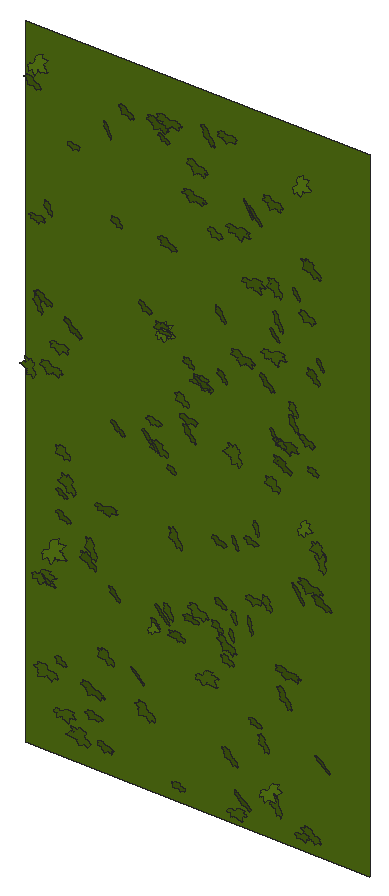
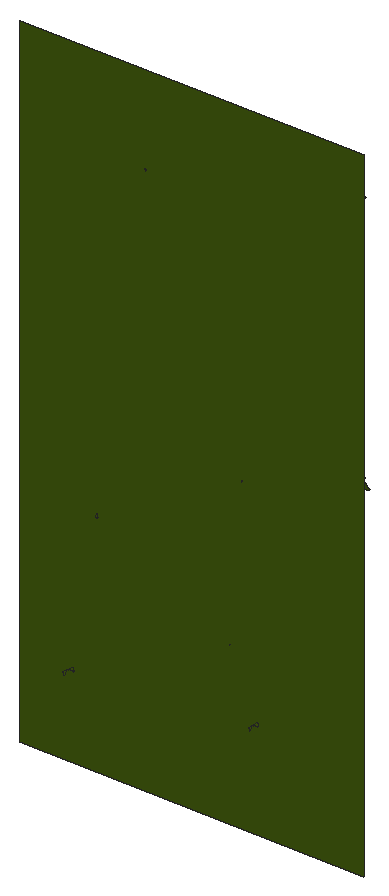
# SketchUp Ruby script. Lengths in inches.
U = 1.inch
M = Sketchup.active_model
def pt(a) = Geom::Point3d.new(a.map { |v| v * U })
def face(e, loops, mat)
  f = e.add_face(loops[0].map { |a| pt(a) })
  loops[1..].each { |l| e.add_face(l.map { |a| pt(a) }).erase! }
  f.material = f.back_material = mat if mat
  f
end
# faces: each face lists its corners as indices into pts; further lists are holes
def faces(e, pts, list, mat = nil) = list.each { |f| face(e, (f[0].is_a?(Array) ? f : [f]).map { |l| l.map { |i| pts[i] } }, mat) }
# xy, xz, yz: faces in a plane at the given z, y or x. An outline is a flat list of corners, or four numbers for a rectangle; further outlines are holes
def ring(l) = l.size == 4 ? [[l[0], l[1]], [l[2], l[1]], [l[2], l[3]], [l[0], l[3]]] : l.each_slice(2).to_a
def flat(e, list, mat, &to3) = list.each { |f| face(e, (f[0].is_a?(Array) ? f : [f]).map { |l| ring(l).map { |u, v| to3.(u, v) } }, mat) }
def xy(e, z, list, mat = nil) = flat(e, list, mat) { |x, y| [x, y, z] }
def xz(e, y, list, mat = nil) = flat(e, list, mat) { |x, z| [x, y, z] }
def yz(e, x, list, mat = nil) = flat(e, list, mat) { |y, z| [x, y, z] }
def lines(e, pts, list) = list.each { |a, b| e.add_line(pt(pts[a]), pt(pts[b])) }
# prism: a flat outline (further loops are holes) pulled along v
def prism(e, loops, v, mat = nil)
  f = face(e, loops, mat); d = Geom::Vector3d.new(v.map { |x| x * U })
  f.pushpull(f.normal.samedirection?(d) ? d.length : -d.length)
end
def box(e, o, s, mat = nil) = prism(e, [[o, [o[0] + s[0], o[1], o[2]], [o[0] + s[0], o[1] + s[1], o[2]], [o[0], o[1] + s[1], o[2]]]], [0, 0, s[2]], mat)
def at(x, y, z, deg = 0) = Geom::Transformation.translation(pt([x, y, z])) * Geom::Transformation.rotation(ORIGIN, Z_AXIS, deg.degrees)
def axes(o, x, y, z) = Geom::Transformation.new([*x, 0, *y, 0, *z, 0, *pt(o).to_a, 1])
def part(name) = M.definitions.add(name)
# library, detail: a bought-in or finely detailed component or shape, given as its bounding box
def library(name, o, s) = part(name).tap { |d| box(d.entities, o, s) }
def detail(e, o, s) = box(e.add_group.entities, o, s)
def put(e, d, t, mat = nil) = e.add_instance(d, t).tap { |i| i.material = mat if mat }
def group(e, t, mat = nil) = e.add_group.tap { |g| g.transformation = t; g.material = mat if mat }.entities
root = M.entities
M.materials.add("[Vegetation Blur 03]").color = [83, 114, 18]
c1 = part("ivy")
xy(c1.entities,0,[[0.782,0,0.786,0,0.787,0.005,0.789,0.009,0.821,0.072,0.875,0.147,1.001,0.272,1.073,0.331,1.137,0.363,1.178,0.379,1.223,0.384,1.272,0.383,1.311,0.374,1.36,0.355,1.399,0.334,1.491,0.285,1.541,0.244,1.583,0.199,1.617,0.15,1.64,0.128,1.662,0.115,1.717,0.105,1.745,0.093,1.784,0.054,1.819,0.057,1.854,0.064,1.882,0.075,1.896,0.074,1.91,0.071,1.937,0.063,1.964,0.053,1.99,0.038,2.016,0.015,2.034,0.002,2.04,0,2.038,0.003,2.036,0.007,2.033,0.038,2.036,0.068,2.045,0.1,2.055,0.116,2.064,0.123,2.077,0.129,2.088,0.129,2.106,0.132,2.118,0.13,2.179,0.132,2.207,0.133,2.225,0.133,2.242,0.138,2.22,0.162,2.207,0.186,2.206,0.213,2.212,0.236,2.228,0.262,2.247,0.274,2.298,0.283,2.355,0.294,2.37,0.296,2.376,0.295,2.377,0.3,2.377,0.303,2.385,0.329,2.411,0.37,2.426,0.392,2.449,0.407,2.511,0.426,2.561,0.444,2.619,0.466,2.589,0.469,2.561,0.476,2.501,0.5,2.449,0.516,2.424,0.523,2.401,0.535,2.377,0.556,2.372,0.568,2.36,0.575,2.268,0.586,2.225,0.592,2.207,0.599,2.194,0.61,2.143,0.65,2.13,0.664,2.122,0.682,2.123,0.7,2.13,0.719,2.148,0.75,2.17,0.781,2.195,0.807,2.221,0.828,2.284,0.874,2.291,0.88,2.288,0.887,2.276,0.9,2.267,0.916,2.265,0.933,2.273,0.967,2.292,1.002,2.313,1.03,2.334,1.054,2.348,1.067,2.358,1.074,2.363,1.076,2.362,1.081,2.35,1.094,2.347,1.11,2.35,1.143,2.359,1.18,2.385,1.254,2.415,1.324,2.448,1.393,2.45,1.4,2.446,1.398,2.44,1.394,2.427,1.383,2.402,1.36,2.376,1.339,2.345,1.324,2.305,1.309,2.282,1.303,2.273,1.306,2.245,1.294,2.212,1.287,2.187,1.291,2.163,1.301,2.142,1.316,2.134,1.327,2.124,1.325,2.09,1.292,2.053,1.259,2.014,1.234,1.973,1.215,1.954,1.21,1.931,1.208,1.909,1.212,1.893,1.22,1.879,1.233,1.872,1.248,1.867,1.281,1.864,1.319,1.821,1.258,1.773,1.197,1.726,1.141,1.698,1.121,1.679,1.116,1.666,1.117,1.647,1.122,1.632,1.129,1.62,1.141,1.617,1.154,1.617,1.219,1.621,1.254,1.623,1.268,1.623,1.281,1.618,1.314,1.606,1.346,1.603,1.375,1.607,1.403,1.603,1.467,1.599,1.499,1.605,1.525,1.614,1.552,1.629,1.577,1.635,1.589,1.629,1.587,1.618,1.582,1.596,1.566,1.581,1.556,1.568,1.552,1.557,1.55,1.545,1.553,1.531,1.562,1.522,1.572,1.504,1.591,1.486,1.611,1.474,1.631,1.457,1.666,1.455,1.684,1.457,1.698,1.452,1.715,1.444,1.728,1.424,1.754,1.419,1.772,1.423,1.786,1.434,1.819,1.444,1.848,1.446,1.855,1.44,1.861,1.43,1.867,1.386,1.904,1.349,1.948,1.326,1.973,1.31,1.995,1.288,2.048,1.284,2.153,1.287,2.254,1.284,2.255,1.282,2.253,1.278,2.247,1.274,2.237,1.266,2.216,1.226,2.125,1.208,2.076,1.184,2.033,1.155,1.984,1.135,1.942,1.111,1.899,1.083,1.861,1.053,1.85,1.059,1.83,1.061,1.809,1.056,1.79,1.049,1.767,1.04,1.749,1.018,1.733,0.994,1.726,0.942,1.734,0.95,1.6875,0.944,1.645,0.932,1.608,0.911,1.585,0.881,1.58,0.854,1.582,0.828,1.588,0.785,1.618,0.773,1.625,0.775,1.614,0.779,1.598,0.796,1.502,0.818,1.402,0.861,1.283,0.882,1.224,0.894,1.174,0.892,1.148,0.886,1.123,0.881,1.107,0.872,1.099,0.849,1.094,0.818,1.092,0.789,1.098,0.762,1.107,0.753,1.113,0.721,1.139,0.698,1.163,0.678,1.194,0.665,1.224,0.628,1.28,0.612,1.312,0.606,1.327,0.606,1.314,0.599,1.282,0.594,1.267,0.581,1.256,0.544,1.245,0.512,1.244,0.473,1.249,0.444,1.256,0.382,1.288,0.339,1.306,0.324,1.316,0.317,1.324,0.309,1.326,0.27,1.314,0.227,1.313,0.185,1.3125,0.152,1.317,0.122,1.328,0.092,1.345,0.073,1.353,0.079,1.338,0.092,1.308,0.117,1.249,0.13,1.215,0.139,1.164,0.147,1.148,0.157,1.136,0.163,1.122,0.174,1.086,0.177,1.067,0.182,1.054,0.186,1.043,0.191,1.038,0.211,1.028,0.237,1.005,0.25,0.974,0.253,0.96,0.25,0.944,0.242,0.914,0.243,0.906,0.249,0.902,0.26,0.894,0.289,0.88,0.307,0.873,0.322,0.862,0.364,0.799,0.403,0.738,0.431,0.709,0.439,0.691,0.441,0.678,0.4375,0.66,0.428,0.645,0.394,0.623,0.303,0.594,0.255,0.581,0.214,0.577,0.179,0.573,0.173,0.568,0.175,0.561,0.167,0.55,0.141,0.523,0.113,0.503,0.077,0.49,0.045,0.486,0.026,0.485,0.019,0.486,0.011,0.483,0,0.471,0.014,0.467,0.044,0.455,0.058,0.447,0.07,0.438,0.097,0.411,0.125,0.394,0.158,0.377,0.174,0.366,0.182,0.359,0.185,0.361,0.242,0.331,0.253,0.316,0.258,0.303,0.262,0.283,0.274,0.278,0.308,0.274,0.341,0.252,0.366,0.226,0.366,0.222,0.37,0.22,0.38,0.221,0.395,0.221,0.425,0.216,0.45,0.207,0.465,0.192,0.473,0.178,0.484,0.15,0.489,0.116,0.483,0.089,0.468,0.058,0.45,0.035,0.435,0.018,0.429,0.011,0.434,0.012,0.438,0.014,0.469,0.019,0.542,0.016,0.581,0.015,0.612,0.027,0.68,0.055,0.696,0.057,0.712,0.052,0.73,0.045,0.741,0.036,0.766,0.014]])
xz(root,174,[[9.54,101,34,147]],"[Vegetation Blur 03]")
put(root,c1,axes([10.7,173.2,126.11],[0.07342,0.0201,-0.45241],[-0.55143,0.12193,-0.05876],[-0.05747,-1.14418,-0.01421]),"[Vegetation Blur 03]")
put(root,c1,axes([10.375,173.2,144.26],[0.33145,0.05992,-0.29685],[-0.36343,0.14447,-0.2657],[-0.03257,-1.00226,-0.05605]),"[Vegetation Blur 03]")
put(root,c1,axes([11.13,173.2,130.26],[0.12192,-0.00071,-0.41999],[-0.49465,0.29998,-0.09572],[-0.14193,-1.04612,-0.02717]),"[Vegetation Blur 03]")
put(root,c1,axes([10.39,173.2,135.43],[0.38883,0.03177,-0.00541],[-0.00902,0.12865,-0.31342],[0.01417,-0.78985,-0.05127]),"[Vegetation Blur 03]")
put(root,c1,axes([10.17,173.2,144.53],[0.22945,0.18892,0.3925],[0.48869,-0.02142,-0.18866],[0.02999,-1.09631,0.07132]),"[Vegetation Blur 03]")
put(root,c1,axes([11.12,173.2,130.72],[0.32489,0.11128,-0.34401],[-0.42351,0.17483,-0.25752],[-0.03505,-1.08109,-0.07706]),"[Vegetation Blur 03]")
put(root,c1,axes([11.22,173.2,107.125],[0.44397,0.1395,-0.34863],[-0.43136,0.05055,-0.3627],[0.03168,-1.26682,-0.05286]),"[Vegetation Blur 03]")
put(root,c1,axes([11.18,173.2,112.72],[0.30297,0.01543,-0.16149],[-0.19571,0.1367,-0.2425],[-0.03016,-0.73198,-0.04869]),"[Vegetation Blur 03]")
put(root,c1,axes([11.8125,173.2,136.52],[0.10541,0.02404,-0.33372],[-0.3979,0.2077,-0.08136],[-0.09494,-0.84377,-0.02954]),"[Vegetation Blur 03]")
put(root,c1,axes([10.42,173.2,112.34],[0.50593,-0.03643,0.3437],[0.41936,0.17969,-0.40818],[0.0424,-1.34262,-0.06395]),"[Vegetation Blur 03]")
put(root,c1,axes([11.39,173.2,126.48],[0.49872,0.09657,-0.2358],[-0.29251,0.12066,-0.4043],[0.0109,-1.17989,-0.06065]),"[Vegetation Blur 03]")
put(root,c1,axes([11.125,173.2,113.75],[0.25598,0.2014,0.48378],[0.59803,0.04143,-0.21349],[0.05748,-1.32803,0.06671]),"[Vegetation Blur 03]")
put(root,c1,axes([11.88,173.2,127.86],[0.50551,0.02715,-0.04471],[-0.05585,0.1053,-0.41049],[0.00753,-1.04102,-0.04269]),"[Vegetation Blur 03]")
put(root,c1,axes([12.46,173.2,107.91],[0.2455,0.02361,-0.20397],[-0.24867,0.10235,-0.19749],[-0.02754,-0.71362,-0.03507]),"[Vegetation Blur 03]")
put(root,c1,axes([12.5,173.2,118.6],[0.23892,0.03876,-0.2007],[-0.24369,0.14566,-0.1888],[-0.038,-0.69034,-0.0511]),"[Vegetation Blur 03]")
put(root,c1,axes([12.77,173.2,121.42],[0.22065,0.07279,-0.34055],[-0.41864,0.06201,-0.17859],[-0.01021,-0.96933,-0.037]),"[Vegetation Blur 03]")
put(root,c1,axes([12.51,173.2,117.24],[0.33471,0.047,-0.24757],[-0.30145,0.17573,-0.26622],[-0.0408,-0.91277,-0.064]),"[Vegetation Blur 03]")
put(root,c1,axes([13.41,173.2,119.6],[0.10808,0.0782,-0.51354],[-0.62715,0.14615,-0.08441],[-0.06373,-1.30565,-0.04021]),"[Vegetation Blur 03]")
put(root,c1,axes([12.05,173.2,104.41],[0.53014,0.02962,0.10212],[0.12282,0.12551,-0.4304],[0.02794,-1.11386,-0.04578]),"[Vegetation Blur 03]")
put(root,c1,axes([12.96,173.2,129.74],[0.55985,-0.09656,-0.30764],[-0.35518,0.35678,-0.44814],[-0.13469,-1.34226,-0.09699]),"[Vegetation Blur 03]")
put(root,c1,axes([13.15,173.2,140.96],[0.30877,0.02964,-0.06253],[-0.07793,0.09874,-0.24894],[0.00225,-0.64717,-0.04084]),"[Vegetation Blur 03]")
put(root,c1,axes([14.29,173.2,103.86],[0.10967,0.16764,-0.53959],[-0.66571,-0.0227,-0.09123],[0.02429,-1.37893,-0.0641]),"[Vegetation Blur 03]")
put(root,c1,axes([14.625,173.2,115.15],[0.17288,0.13727,-0.46997],[-0.57483,0.20036,-0.13164],[-0.0749,-1.22089,-0.07445]),"[Vegetation Blur 03]")
put(root,c1,axes([14.32,173.2,107.03],[0.53027,0.09687,-0.32245],[-0.39653,0.24084,-0.42296],[-0.03295,-1.33931,-0.09938]),"[Vegetation Blur 03]")
put(root,c1,axes([14.89,173.2,116.17],[0.24952,-0.09563,-0.45788],[-0.54485,0.27669,-0.20686],[-0.14163,-1.23287,-0.01091]),"[Vegetation Blur 03]")
put(root,c1,axes([14.68,173.2,105.23],[0.30579,0.15468,-0.23311],[-0.2938,0.07258,-0.24913],[0.03027,-0.858,-0.0631]),"[Vegetation Blur 03]")
put(root,c1,axes([15.8,173.2,109.51],[0.24902,0.09318,-0.40988],[-0.50306,0.12516,-0.1991],[-0.03467,-1.14673,-0.05504]),"[Vegetation Blur 03]")
put(root,c1,axes([15.92,173.2,142.97],[0.14161,0.02749,-0.37414],[-0.43235,0.33737,-0.1051],[-0.153,-0.92792,-0.0493]),"[Vegetation Blur 03]")
put(root,c1,axes([15.29,173.2,103.54],[0.43132,0.00683,-0.12215],[-0.14822,0.15148,-0.34728],[-0.02104,-0.9272,-0.05763]),"[Vegetation Blur 03]")
put(root,c1,axes([14.98,173.2,118.54],[0.54712,0.06533,0.00829],[0.00324,0.23778,-0.43729],[0.03318,-1.10066,-0.09398]),"[Vegetation Blur 03]")
put(root,c1,axes([16.35,173.2,113.58],[0.21131,0.04206,-0.34485],[-0.41038,0.25638,-0.16258],[-0.10272,-0.93777,-0.05992]),"[Vegetation Blur 03]")
put(root,c1,axes([16.72,173.2,137.26],[0.07231,0.11382,-0.30015],[-0.37128,0.06711,-0.05557],[-0.02172,-0.76837,-0.04931]),"[Vegetation Blur 03]")
put(root,c1,axes([16.36,173.2,124.3],[0.37381,-0.01776,-0.27785],[-0.3272,0.26974,-0.29592],[-0.09444,-1.00486,-0.07453]),"[Vegetation Blur 03]")
put(root,c1,axes([17.05,173.2,144.67],[0.32569,0.04627,-0.29452],[-0.35796,0.18221,-0.25916],[-0.05099,-0.98359,-0.06186]),"[Vegetation Blur 03]")
put(root,c1,axes([18.04,173.2,108.76],[0.09506,0.21771,-0.46057],[-0.55663,0.32363,-0.05246],[-0.14082,-1.13231,-0.10355]),"[Vegetation Blur 03]")
put(root,c1,axes([18.39,173.2,107.16],[0.44315,0.00145,-0.39097],[-0.47521,0.17095,-0.35867],[-0.06051,-1.33197,-0.04646]),"[Vegetation Blur 03]")
put(root,c1,axes([18.33,173.2,132.65],[0.35037,-0.01321,-0.20166],[-0.24181,0.16441,-0.28153],[-0.0512,-0.86678,-0.05033]),"[Vegetation Blur 03]")
put(root,c1,axes([18.6,173.2,124.47],[0.46716,-0.062,-0.38996],[-0.44887,0.42109,-0.3687],[-0.16652,-1.30905,-0.10013]),"[Vegetation Blur 03]")
put(root,c1,axes([18.96,173.2,125.49],[0.29858,0.09929,-0.17499],[-0.21887,0.06675,-0.24279],[0.01995,-0.75348,-0.04457]),"[Vegetation Blur 03]")
put(root,c1,axes([19.34,173.2,112.61],[0.12889,0.05373,-0.25764],[-0.31029,0.16238,-0.09807],[-0.06367,-0.68262,-0.04361]),"[Vegetation Blur 03]")
put(root,c1,axes([18.82,173.2,111.65],[0.07011,0.12287,0.23012],[0.28735,0.0166,-0.05971],[0.0224,-0.59768,0.04565]),"[Vegetation Blur 03]")
put(root,c1,axes([19.65,173.2,124.09],[0.19085,0.16255,-0.44019],[-0.54494,0.0863,-0.15236],[-0.01363,-1.17416,-0.07214]),"[Vegetation Blur 03]")
put(root,c1,axes([18.97,173.2,144.74],[0.51903,0.05216,-0.26245],[-0.32095,0.20906,-0.41624],[-0.03231,-1.23893,-0.08129]),"[Vegetation Blur 03]")
put(root,c1,axes([19.49,173.2,113.64],[0.40831,-0.04926,-0.36189],[-0.41615,0.39004,-0.3211],[-0.15494,-1.17746,-0.09123]),"[Vegetation Blur 03]")
put(root,c1,axes([20.12,173.2,131.72],[0.10531,0.2061,-0.4524],[-0.56328,0.04564,-0.08406],[-0.00345,-1.16018,-0.08367]),"[Vegetation Blur 03]")
put(root,c1,axes([19.73,173.2,143.77],[0.26625,0.02526,-0.1848],[-0.22371,0.14694,-0.21152],[-0.03714,-0.70407,-0.05077]),"[Vegetation Blur 03]")
put(root,c1,axes([19.9375,173.2,137.28],[0.33022,0.14446,-0.3444],[-0.42741,0.15711,-0.26261],[-0.01782,-1.09139,-0.08339]),"[Vegetation Blur 03]")
put(root,c1,axes([19.58,173.2,131.2],[0.33133,0.03179,-0.00697],[-0.01113,0.11989,-0.26643],[0.0137,-0.67142,-0.0479]),"[Vegetation Blur 03]")
put(root,c1,axes([19.52,173.2,145.05],[0.59461,0.12109,-0.18026],[-0.22736,0.18289,-0.48022],[0.02354,-1.29241,-0.08484]),"[Vegetation Blur 03]")
put(root,c1,axes([19.37,173.2,130.58],[0.10294,0.13872,0.40661],[0.50198,0.02961,-0.08624],[0.02785,-1.04645,0.05146]),"[Vegetation Blur 03]")
put(root,c1,axes([20.3,173.2,113.9],[0.21141,-0.03642,-0.34067],[-0.40654,0.204,-0.17147],[-0.09632,-0.94099,-0.02399]),"[Vegetation Blur 03]")
put(root,c1,axes([20.64,173.2,122.76],[0.04516,0.08728,-0.24004],[-0.29622,0.06188,-0.03358],[-0.02362,-0.6092,-0.0378]),"[Vegetation Blur 03]")
put(root,c1,axes([20.77,173.2,118.9375],[0.2944,-0.05147,-0.44172],[-0.52796,0.2576,-0.2391],[-0.12176,-1.24142,-0.0313]),"[Vegetation Blur 03]")
put(root,c1,axes([20.98,173.2,112.41],[0.11047,0.20453,-0.35161],[-0.44126,-0.0065,-0.09294],[0.02783,-0.9152,-0.07792]),"[Vegetation Blur 03]")
put(root,c1,axes([20.93,173.2,102.8125],[0.1696,0.1381,-0.24942],[-0.31204,0.02191,-0.13942],[0.02307,-0.7189,-0.05216]),"[Vegetation Blur 03]")
put(root,c1,axes([21.25,173.2,127.74],[0.21346,0.05085,-0.33078],[-0.40485,0.09932,-0.17162],[-0.03132,-0.93739,-0.03613]),"[Vegetation Blur 03]")
put(root,c1,axes([21.67,173.2,125.78],[0.25339,0.01902,-0.3994],[-0.47391,0.29322,-0.19806],[-0.12245,-1.09547,-0.05995]),"[Vegetation Blur 03]")
put(root,c1,axes([21.18,173.2,126.45],[0.41502,0.09791,-0.15811],[-0.19925,0.15826,-0.33295],[0.0098,-0.92912,-0.07337]),"[Vegetation Blur 03]")
put(root,c1,axes([21.83,173.2,130.08],[0.09179,0.09251,-0.29251],[-0.35994,0.08732,-0.07089],[-0.03033,-0.7563,-0.04396]),"[Vegetation Blur 03]")
put(root,c1,axes([21.78,173.2,113.8],[0.1902,0.17643,-0.26649],[-0.33646,0.03567,-0.15623],[0.02775,-0.7768,-0.0677]),"[Vegetation Blur 03]")
put(root,c1,axes([21.55,173.2,140.93],[0.48948,0.16058,-0.27855],[-0.34964,0.16113,-0.39462],[0.01829,-1.21733,-0.08898]),"[Vegetation Blur 03]")
put(root,c1,axes([21.79,173.2,142.97],[0.53586,0.00327,-0.21137],[-0.25728,0.14717,-0.4341],[-0.0297,-1.21585,-0.05311]),"[Vegetation Blur 03]")
put(root,c1,axes([21.99,173.2,114.7],[0.47827,0.03325,-0.27343],[-0.33498,0.10885,-0.38819],[-0.01718,-1.19669,-0.04291]),"[Vegetation Blur 03]")
put(root,c1,axes([22.98,173.2,129.36],[0.08849,0.22325,-0.50781],[-0.6312,-0.01504,-0.0743],[0.02262,-1.29319,-0.0868]),"[Vegetation Blur 03]")
put(root,c1,axes([22.13,173.2,129.14],[0.46406,-0.05319,-0.06714],[-0.07481,0.21257,-0.37089],[-0.04289,-0.94624,-0.07954]),"[Vegetation Blur 03]")
put(root,c1,axes([22.91,173.2,145.39],[0.37946,-0.0754,-0.40939],[-0.47883,0.34147,-0.30552],[-0.15388,-1.24846,-0.05884]),"[Vegetation Blur 03]")
put(root,c1,axes([22.06,173.2,109.94],[0.46309,-0.00814,0.32802],[0.3991,0.15897,-0.37467],[0.04767,-1.25175,-0.04972]),"[Vegetation Blur 03]")
put(root,c1,axes([23.37,173.2,139.09],[0.32097,0.04197,-0.19874],[-0.24426,0.07998,-0.2601],[-0.00735,-0.82521,-0.03532]),"[Vegetation Blur 03]")
put(root,c1,axes([23.76,173.2,114.05],[0.16976,0.07158,-0.29867],[-0.3654,0.12339,-0.13369],[-0.04012,-0.82092,-0.04613]),"[Vegetation Blur 03]")
put(root,c1,axes([24,173.2,134.07],[0.15729,0.04975,-0.38701],[-0.46067,0.26502,-0.11935],[-0.11503,-0.99334,-0.05122]),"[Vegetation Blur 03]")
put(root,c1,axes([23.51,173.2,119.48],[0.35115,0.05857,-0.18722],[-0.23024,0.1649,-0.27952],[-0.02054,-0.84722,-0.06735]),"[Vegetation Blur 03]")
put(root,c1,axes([23.92,173.2,115.54],[0.17674,0.08976,-0.26223],[-0.3229,0.11764,-0.13863],[-0.02967,-0.7454,-0.05345]),"[Vegetation Blur 03]")
put(root,c1,axes([24.2,173.2,130.0625],[0.08767,0.08949,-0.34433],[-0.41588,0.19217,-0.06267],[-0.08326,-0.86566,-0.04951]),"[Vegetation Blur 03]")
put(root,c1,axes([23.98,173.2,113.4],[0.54219,-0.07189,-0.27942],[-0.3337,0.21166,-0.43986],[-0.08416,-1.30245,-0.05606]),"[Vegetation Blur 03]")
put(root,c1,axes([23.85,173.2,145.41],[0.46012,0.08661,-0.09796],[-0.12471,0.12465,-0.37281],[0.02504,-0.97055,-0.05662]),"[Vegetation Blur 03]")
put(root,c1,axes([24.37,173.2,112.17],[0.24584,0.04332,-0.24097],[-0.29547,0.08344,-0.19842],[-0.01781,-0.78621,-0.03434]),"[Vegetation Blur 03]")
put(root,c1,axes([24.46,173.2,106.26],[0.33588,0.02262,-0.39753],[-0.47681,0.26549,-0.26596],[-0.10014,-1.18823,-0.067]),"[Vegetation Blur 03]")
put(root,c1,axes([24.9,173.2,113.78],[0.07952,-0.02515,-0.25316],[-0.29832,0.17612,-0.06516],[-0.08589,-0.63499,-0.00805]),"[Vegetation Blur 03]")
put(root,c1,axes([25.32,173.2,125.72],[0.10377,0.02186,-0.53621],[-0.65451,0.12482,-0.08356],[-0.05827,-1.36305,-0.01625]),"[Vegetation Blur 03]")
put(root,c1,axes([25.11,173.2,114.94],[0.04974,-0.00028,-0.27725],[-0.32677,0.19308,-0.03908],[-0.09286,-0.67961,-0.01099]),"[Vegetation Blur 03]")
put(root,c1,axes([25,173.2,119.85],[0.19183,-0.05588,-0.2698],[-0.31224,0.23474,-0.15552],[-0.11192,-0.75067,-0.02855]),"[Vegetation Blur 03]")
put(root,c1,axes([24.39,173.2,102.32],[0.46585,0.02288,0.14137],[0.17091,0.11775,-0.37813],[0.0303,-1.01595,-0.04064]),"[Vegetation Blur 03]")
put(root,c1,axes([24.34,173.2,139.67],[0.63593,0.00439,0.02808],[0.0337,0.19557,-0.51321],[0.00724,-1.29586,-0.07736]),"[Vegetation Blur 03]")
put(root,c1,axes([24.875,173.2,131.9375],[0.61818,0.02753,-0.20694],[-0.25253,0.20999,-0.49806],[-0.0265,-1.35881,-0.08116]),"[Vegetation Blur 03]")
put(root,c1,axes([25.03,173.2,103.77],[0.53938,-0.11783,-0.24861],[-0.28048,0.34993,-0.43141],[-0.13192,-1.22575,-0.09926]),"[Vegetation Blur 03]")
put(root,c1,axes([25.9375,173.2,141.38],[0.10747,0.09693,-0.42949],[-0.50045,0.37307,-0.07017],[-0.16944,-1.0404,-0.06517]),"[Vegetation Blur 03]")
put(root,c1,axes([26.19,173.2,114.9],[0.06026,0.01776,-0.40154],[-0.46093,0.35917,-0.04358],[-0.17229,-0.95467,-0.02387]),"[Vegetation Blur 03]")
put(root,c1,axes([25.91,173.2,120.24],[0.26692,0.10027,-0.19485],[-0.24358,0.09015,-0.21495],[0.00657,-0.73139,-0.05321]),"[Vegetation Blur 03]")
put(root,c1,axes([25.875,173.2,116.51],[0.38415,0.08832,-0.09325],[-0.11924,0.10565,-0.31143],[0.02608,-0.81794,-0.0503]),"[Vegetation Blur 03]")
put(root,c1,axes([26.125,173.2,141.38],[0.42548,-0.09437,-0.33716],[-0.38139,0.39508,-0.33797],[-0.16527,-1.15464,-0.08808]),"[Vegetation Blur 03]")
put(root,c1,axes([26.3125,173.2,108.8],[0.21856,0.08137,-0.22546],[-0.27868,0.10188,-0.17416],[-0.01478,-0.71768,-0.05028]),"[Vegetation Blur 03]")
put(root,c1,axes([26.66,173.2,121.25],[0.07886,-0.02245,-0.3122],[-0.36365,0.24601,-0.06396],[-0.11923,-0.76517,-0.0114]),"[Vegetation Blur 03]")
put(root,c1,axes([25.42,173.2,136.53],[0.5764,-0.04158,0.19028],[0.23362,0.17732,-0.46527],[0.01378,-1.26714,-0.07135]),"[Vegetation Blur 03]")
put(root,c1,axes([27,173.2,107.95],[0.28434,-0.07307,-0.35446],[-0.41994,0.239,-0.23213],[-0.11635,-1.04116,-0.02841]),"[Vegetation Blur 03]")
put(root,c1,axes([27.44,173.2,116.83],[0.12874,0.00958,-0.35889],[-0.43298,0.16781,-0.10275],[-0.07698,-0.92784,-0.02229]),"[Vegetation Blur 03]")
put(root,c1,axes([26.94,173.2,131.04],[0.44147,-0.0788,-0.2903],[-0.33877,0.28169,-0.35517],[-0.11502,-1.13213,-0.06817]),"[Vegetation Blur 03]")
put(root,c1,axes([27.84,173.2,124.625],[0.1471,0.09742,-0.39347],[-0.48397,0.0748,-0.1176],[-0.02114,-1.03455,-0.04555]),"[Vegetation Blur 03]")
put(root,c1,axes([27.15,173.2,142.52],[0.51764,0.02568,-0.18283],[-0.22378,0.14257,-0.41887],[-0.01616,-1.15189,-0.05592]),"[Vegetation Blur 03]")
put(root,c1,axes([26.68,173.2,104.1],[0.37101,0.18964,0.31894],[0.39968,-0.06988,-0.30314],[0.03834,-1.10666,0.0738]),"[Vegetation Blur 03]")
put(root,c1,axes([28.01,173.2,137.29],[0.18125,0.04011,-0.45454],[-0.55361,0.15105,-0.14494],[-0.06386,-1.19573,-0.03356]),"[Vegetation Blur 03]")
put(root,c1,axes([27.66,173.2,134.11],[0.28115,-0.04858,-0.24392],[-0.28246,0.2397,-0.22437],[-0.10049,-0.80964,-0.05179]),"[Vegetation Blur 03]")
put(root,c1,axes([27.69,173.2,127.74],[0.24639,-0.0769,-0.23479],[-0.27054,0.21951,-0.20041],[-0.10474,-0.7479,-0.03468]),"[Vegetation Blur 03]")
put(root,c1,axes([27.98,173.2,104.45],[0.27997,-0.09905,-0.45822],[-0.54252,0.30141,-0.23104],[-0.15235,-1.25535,-0.01932]),"[Vegetation Blur 03]")
put(root,c1,axes([26.84,173.2,132.5],[0.59787,0.07047,0.08314],[0.09735,0.14687,-0.48587],[0.04553,-1.23935,-0.05285]),"[Vegetation Blur 03]")
put(root,c1,axes([28.4375,173.2,126.04],[0.15268,0.21133,-0.48982],[-0.60568,0.18355,-0.11329],[-0.06257,-1.26109,-0.09857]),"[Vegetation Blur 03]")
put(root,c1,axes([27.97,173.2,135.32],[0.36249,-0.1648,-0.3565],[-0.41016,0.32061,-0.3011],[-0.17026,-1.12322,-0.03364]),"[Vegetation Blur 03]")
put(root,c1,axes([28.33,173.2,127.25],[0.13027,0.06294,-0.24641],[-0.30303,0.06322,-0.10416],[-0.01626,-0.67369,-0.0328]),"[Vegetation Blur 03]")
put(root,c1,axes([28.34,173.2,111.5625],[0.44681,-0.13861,-0.40686],[-0.47518,0.33403,-0.36549],[-0.1651,-1.33648,-0.04915]),"[Vegetation Blur 03]")
put(root,c1,axes([28.01,173.2,112.84],[0.5883,0.12569,-0.22776],[-0.28567,0.25569,-0.4693],[0.00068,-1.31528,-0.113]),"[Vegetation Blur 03]")
put(root,c1,axes([27.67,173.2,127.23],[0.67545,-0.01499,0.0047],[0.00705,0.26519,-0.54115],[-0.00605,-1.36446,-0.10523]),"[Vegetation Blur 03]")
put(root,c1,axes([29.55,173.2,118.12],[0.10735,0.13666,-0.49936],[-0.59338,0.3622,-0.06937],[-0.16335,-1.22594,-0.07616]),"[Vegetation Blur 03]")
put(root,c1,axes([29.12,173.2,129.08],[0.29122,-0.09132,-0.34949],[-0.40801,0.28097,-0.238],[-0.13739,-1.02797,-0.034]),"[Vegetation Blur 03]")
put(root,c1,axes([29.26,173.2,129.86],[0.15958,-0.02123,-0.31626],[-0.37905,0.17205,-0.12921],[-0.08118,-0.84504,-0.01836]),"[Vegetation Blur 03]")
put(root,c1,axes([29.33,173.2,137.21],[0.19632,-0.0358,-0.23719],[-0.2774,0.19596,-0.15758],[-0.08838,-0.69459,-0.03223]),"[Vegetation Blur 03]")
put(root,c1,axes([29.07,173.2,143.25],[0.0857,0.17777,0.39101],[0.48593,0.02942,-0.07304],[0.02949,-1.0011,0.06729]),"[Vegetation Blur 03]")
put(root,c1,axes([29.25,173.2,102.52],[0.36983,0.02306,0.04655],[0.05424,0.13467,-0.29755],[0.02088,-0.75816,-0.05144]),"[Vegetation Blur 03]")
put(root,c1,axes([29.46,173.2,121.63],[0.07333,0.12212,0.31359],[0.38829,0.01811,-0.06159],[0.01986,-0.80476,0.0462]),"[Vegetation Blur 03]")
put(root,c1,axes([29.73,173.2,128.12],[0.41941,-0.00434,-0.1684],[-0.2031,0.16133,-0.33757],[-0.03648,-0.94822,-0.05667]),"[Vegetation Blur 03]")
put(root,c1,axes([29.82,173.2,136.09],[0.40291,0.01111,-0.21009],[-0.25613,0.11786,-0.3262],[-0.02632,-0.9768,-0.04175]),"[Vegetation Blur 03]")
put(root,c1,axes([30.35,173.2,139.4],[0.2991,0.11532,-0.48246],[-0.59082,0.19391,-0.23668],[-0.05934,-1.34945,-0.07524]),"[Vegetation Blur 03]")
put(root,c1,axes([29.72,173.2,118.99],[0.56725,0.10726,-0.27566],[-0.34171,0.20149,-0.45603],[-0.00596,-1.34353,-0.0904]),"[Vegetation Blur 03]")
put(root,c1,axes([30.23,173.2,103.27],[0.36107,0.086,-0.36328],[-0.44668,0.11955,-0.29126],[-0.01905,-1.17336,-0.0563]),"[Vegetation Blur 03]")
put(root,c1,axes([30.71,173.2,132.39],[0.11247,0.10768,-0.41349],[-0.50254,0.19726,-0.08297],[-0.08291,-1.04957,-0.05801]),"[Vegetation Blur 03]")
put(root,c1,axes([30.67,173.2,126.21],[0.08326,0.10722,-0.24971],[-0.31037,0.02564,-0.0672],[0.00148,-0.65202,-0.0437]),"[Vegetation Blur 03]")
put(root,c1,axes([31.15,173.2,107.78],[0.15704,0.2136,-0.46973],[-0.57168,0.3147,-0.1048],[-0.12334,-1.18664,-0.11235]),"[Vegetation Blur 03]")
put(root,c1,axes([31.08,173.2,121.61],[0.20248,0.05039,-0.42079],[-0.51446,0.11243,-0.16277],[-0.042,-1.13431,-0.03483]),"[Vegetation Blur 03]")
put(root,c1,axes([31.125,173.2,133.18],[0.08292,0.05054,-0.29306],[-0.34577,0.22171,-0.05915],[-0.09993,-0.72524,-0.0385]),"[Vegetation Blur 03]")
put(root,c1,axes([30.95,173.2,118.22],[0.33518,0.12814,-0.38098],[-0.46864,0.20726,-0.26366],[-0.04654,-1.16428,-0.08887]),"[Vegetation Blur 03]")
put(root,c1,axes([31.45,173.2,121.03],[0.10156,-0.07064,-0.4993],[-0.59327,0.30784,-0.08723],[-0.15326,-1.23847,0.0068]),"[Vegetation Blur 03]")
